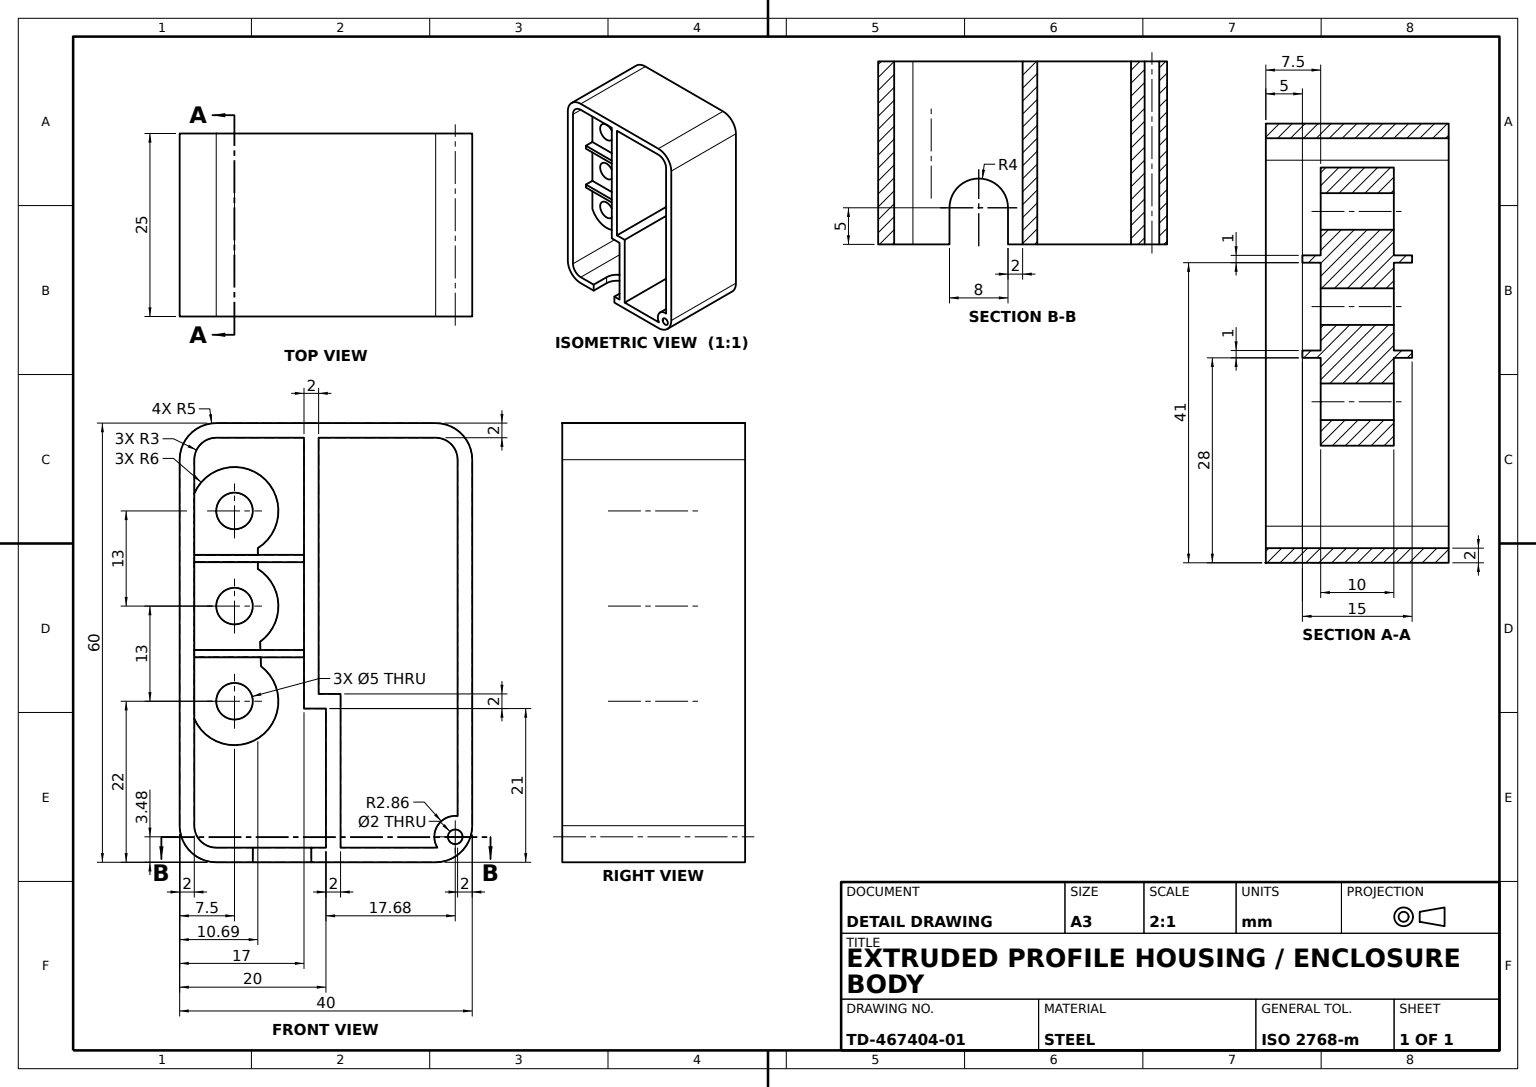
solid
v1 (-3,-9,12.5)
v2 (-3,-9,-12.5)
e1 v1 v2 LINE
v3 (0,-9,-12.5)
e2 v2 v3 LINE
v4 (0,-9,12.5)
e3 v4 v3 LINE
e4 v1 v4 LINE
face PLANE(AX(P(0,-9,12.5),D(0,1,0),D(0,0,1))) rev [e1 e2 -e3 -e4]
v5 (-10,-30,7.5)
v6 (-10,-30,12.5)
e5 v5 v6 LINE
v7 (-10,-28,7.5)
e6 v7 v5 LINE
v8 (-10,-28,12.5)
e7 v7 v8 LINE
e8 v8 v6 LINE
face PLANE(AX(P(-10,-30.000012,0),D(-1,0,0),D(0,0,1))) rev [-e5 -e6 e7 e8]
v9 (-9.3124,12.915793,5)
v10 (-18,20.396936,5)
e9 v9 v10 CIRCLE(AX(P(-12.5,17.99902,5),D(0,0,1),D(1,0,0)),6)
v11 (-18,11.99902,5)
e10 v10 v11 LINE
v12 (-9.3124,11.99902,5)
e11 v11 v12 LINE
e12 v9 v12 LINE
v13 (-10,17.99902,5)
v14 (-15,17.99902,5)
e13 v13 v14 CIRCLE(AX(P(-12.5,17.99902,5),D(0,0,1),D(1,0,0)),2.5)
e14 v14 v13 CIRCLE(AX(P(-12.5,17.99902,5),D(0,0,1),D(1,0,0)),2.5)
face PLANE(AX(P(0,0,5),D(0,0,1),D(1,0,0))) [e9 e10 e11 -e12] [-e13 -e14]
v15 (-10,4.99902,5)
v16 (-15,4.99902,5)
e15 v15 v16 CIRCLE(AX(P(-12.5,4.99902,5),D(0,0,1),D(1,0,0)),2.5)
e16 v16 v15 CIRCLE(AX(P(-12.5,4.99902,5),D(0,0,1),D(1,0,0)),2.5)
v17 (-9.3124,10.99902,5)
v18 (-9.3124,10.082248,5)
e17 v17 v18 LINE
v19 (-18,10.99902,5)
e18 v19 v17 LINE
v20 (-18,-1.00098,5)
e19 v19 v20 LINE
v21 (-8.958313,-1.00098,5)
e20 v20 v21 LINE
v22 (-8.994852,0.129325,5)
e21 v22 v21 LINE
e22 v22 v18 CIRCLE(AX(P(-12.5,4.99902,5),D(0,0,1),D(1,0,0)),6)
face PLANE(AX(P(0,0,5),D(0,0,1),D(1,0,0))) [-e15 -e16] [-e17 -e18 e19 e20 -e21 e22]
v23 (-6,-28,3.5)
v24 (-6,-30,3.5)
e23 v23 v24 LINE
v25 (-2,-30,7.5)
e24 v25 v24 CIRCLE(AX(P(-6,-30,7.5),D(0,1,0),D(0,0,-1)),4)
v26 (-2,-28,7.5)
e25 v26 v25 LINE
e26 v23 v26 CIRCLE(AX(P(-6,-28,7.5),D(0,-1,0),D(0,0,1)),4)
face CYL(AX(P(-6,-26,7.5),D(0,-1,0),D(0,0,-1)),4) rev [e23 -e24 -e25 -e26]
v27 (-3,-1.00098,7.5)
v28 (-3,-1.00098,-7.5)
e27 v27 v28 LINE
v29 (-18,-1.00098,-7.5)
e28 v29 v28 LINE
v30 (-18,-1.00098,-5)
e29 v30 v29 LINE
v31 (-8.958313,-1.00098,-5)
e30 v30 v31 LINE
e31 v21 v31 LINE
v32 (-18,-1.00098,7.5)
e32 v32 v20 LINE
e33 v32 v27 LINE
face PLANE(AX(P(0,-1.00098,7.5),D(0,1,0),D(0,0,1))) [e27 -e28 -e29 e30 -e31 -e20 -e32 e33]
v33 (-8.994852,0.129325,-5)
v34 (-9.3124,10.082248,-5)
e34 v33 v34 CIRCLE(AX(P(-12.5,4.99902,-5),D(0,0,1),D(1,0,0)),6)
e35 v18 v34 LINE
e36 v22 v33 LINE
face CYL(AX(P(-12.5,4.99902,5),D(0,0,-1),D(-1,0,0)),6) [e34 -e35 -e22 e36]
v35 (-18,10.99902,-5)
e37 v35 v30 LINE
v36 (-18,-2.00098,-7.5)
e38 v29 v36 LINE
v37 (-18,-2.00098,-5)
e39 v37 v36 LINE
v38 (-18,-10.398895,-5)
e40 v37 v38 LINE
v39 (-18,-10.398895,5)
e41 v39 v38 LINE
v40 (-18,-2.00098,5)
e42 v40 v39 LINE
v41 (-18,-2.00098,7.5)
e43 v41 v40 LINE
e44 v32 v41 LINE
v42 (-18,10.99902,7.5)
e45 v42 v19 LINE
v43 (-18,11.99902,7.5)
e46 v43 v42 LINE
e47 v43 v11 LINE
v44 (-18,20.396936,-5)
e48 v10 v44 LINE
v45 (-18,11.99902,-5)
e49 v44 v45 LINE
v46 (-18,11.99902,-7.5)
e50 v45 v46 LINE
v47 (-18,10.99902,-7.5)
e51 v46 v47 LINE
e52 v35 v47 LINE
v48 (-18,25,12.5)
v49 (-18,25,-12.5)
e53 v48 v49 LINE
v50 (-18,-25,12.5)
e54 v48 v50 LINE
v51 (-18,-25,-12.5)
e55 v50 v51 LINE
e56 v49 v51 LINE
face PLANE(AX(P(-18,0,12.5),D(1,0,0),D(0,1,0))) [e37 e29 e38 -e39 e40 -e41 -e42 -e43 -e44 e32 -e19 -e45 -e46 e47 -e10 e48 e49 e50 e51 -e52] [-e53 e54 e55 -e56]
v52 (-2,-28,12.5)
e57 v52 v26 LINE
v53 (0,-28,12.5)
e58 v52 v53 LINE
v54 (0,-28,-12.5)
e59 v53 v54 LINE
v55 (-15,-28,-12.5)
e60 v55 v54 LINE
v56 (-15,-28,12.5)
e61 v56 v55 LINE
e62 v56 v8 LINE
e63 v7 v23 CIRCLE(AX(P(-6,-28,7.5),D(0,-1,0),D(0,0,1)),4)
face PLANE(AX(P(0,-28,12.5),D(0,1,0),D(0,0,1))) [e26 -e57 e58 e59 -e60 -e61 e62 -e7 e63]
v57 (-3,-2.00098,7.5)
e64 v41 v57 LINE
e65 v27 v57 LINE
face PLANE(AX(P(0,0,7.5),D(0,0,1),D(1,0,0))) [e44 e64 -e65 -e33]
v58 (15,30,12.5)
v59 (15,30,-12.5)
e66 v58 v59 LINE
v60 (-15,30,-12.5)
e67 v60 v59 LINE
v61 (-15,30,12.5)
e68 v61 v60 LINE
e69 v61 v58 LINE
face PLANE(AX(P(0,30,12.5),D(0,1,0),D(0,0,1))) [e66 -e67 -e68 e69]
v62 (18.679633,-26.51945,12.5)
v63 (18.679633,-26.51945,-12.5)
e70 v62 v63 LINE
v64 (16.679633,-26.51945,12.5)
e71 v62 v64 CIRCLE(AX(P(17.679633,-26.51945,12.5),D(0,0,1),D(1,0,0)),1)
v65 (16.679633,-26.51945,-12.5)
e72 v64 v65 LINE
e73 v63 v65 CIRCLE(AX(P(17.679633,-26.51945,-12.5),D(0,0,1),D(1,0,0)),1)
face CYL(AX(P(17.679633,-26.51945,12.5),D(0,0,-1),D(-1,0,0)),1) rev [-e70 e71 e72 -e73]
v66 (-15,17.99902,-5)
e74 v14 v66 LINE
v67 (-10,17.99902,-5)
e75 v13 v67 LINE
e76 v66 v67 CIRCLE(AX(P(-12.5,17.99902,-5),D(0,0,1),D(1,0,0)),2.5)
face CYL(AX(P(-12.5,17.99902,5),D(0,0,-1),D(-1,0,0)),2.5) rev [-e74 e14 e75 -e76]
v68 (-20,25,12.5)
v69 (-20,25,-12.5)
e77 v68 v69 LINE
v70 (-20,-25,-12.5)
e78 v69 v70 LINE
v71 (-20,-25,12.5)
e79 v71 v70 LINE
e80 v68 v71 LINE
face PLANE(AX(P(-20,0,12.5),D(1,0,0),D(0,1,0))) rev [e77 e78 -e79 -e80]
v72 (-8.886875,-3.210851,5)
v73 (-8.886875,-3.210851,-5)
e81 v72 v73 LINE
e82 v39 v72 CIRCLE(AX(P(-12.5,-8.00098,5),D(0,0,1),D(1,0,0)),6)
e83 v38 v73 CIRCLE(AX(P(-12.5,-8.00098,-5),D(0,0,1),D(1,0,0)),6)
face CYL(AX(P(-12.5,-8.00098,5),D(0,0,-1),D(-1,0,0)),6) [-e81 -e82 e41 e83]
v74 (-3,-2.00098,-7.5)
e84 v28 v74 LINE
e85 v36 v74 LINE
face PLANE(AX(P(0,0,-7.5),D(0,0,1),D(1,0,0))) rev [e28 e84 -e85 -e38]
v75 (14.8185,-26.51945,12.5)
v76 (14.8185,-26.51945,-12.5)
e86 v75 v76 LINE
v77 (15.231357,-28,-12.5)
e87 v76 v77 CIRCLE(AX(P(17.679633,-26.51945,-12.5),D(0,0,1),D(1,0,0)),2.861134)
v78 (15.231357,-28,12.5)
e88 v78 v77 LINE
e89 v75 v78 CIRCLE(AX(P(17.679633,-26.51945,12.5),D(0,0,1),D(1,0,0)),2.861134)
face CYL(AX(P(17.679633,-26.51945,12.5),D(0,0,-1),D(-1,0,0)),2.861134) [e86 e87 -e88 -e89]
v79 (-1,28,12.5)
v80 (-1,28,-12.5)
e90 v79 v80 LINE
v81 (15,28,-12.5)
e91 v80 v81 LINE
v82 (15,28,12.5)
e92 v82 v81 LINE
e93 v79 v82 LINE
face PLANE(AX(P(0,28,12.5),D(0,1,0),D(0,0,1))) rev [e90 e91 -e92 -e93]
e94 v60 v69 CIRCLE(AX(P(-15,25,-12.5),D(0,0,1),D(1,0,0)),5)
v83 (20,25,-12.5)
e95 v59 v83 CIRCLE(AX(P(15,25,-12.5),D(0,0,-1),D(1,0,0)),5)
v84 (20,-25,-12.5)
e96 v83 v84 LINE
v85 (15,-30,-12.5)
e97 v85 v84 CIRCLE(AX(P(15,-25,-12.5),D(0,0,1),D(1,0,0)),5)
v86 (-15,-30,-12.5)
e98 v86 v85 LINE
e99 v70 v86 CIRCLE(AX(P(-15,-25,-12.5),D(0,0,1),D(1,0,0)),5)
v87 (18,25,-12.5)
e100 v81 v87 CIRCLE(AX(P(15,25,-12.5),D(0,0,-1),D(1,0,0)),3)
v88 (-1,-7,-12.5)
e101 v80 v88 LINE
v89 (2,-7,-12.5)
e102 v88 v89 LINE
v90 (2,-28,-12.5)
e103 v89 v90 LINE
e104 v90 v77 LINE
v91 (18,-23.676309,-12.5)
e105 v91 v76 CIRCLE(AX(P(17.679633,-26.51945,-12.5),D(0,0,1),D(1,0,0)),2.861134)
e106 v87 v91 LINE
v92 (-15,28,-12.5)
v93 (-3,28,-12.5)
e107 v92 v93 LINE
e108 v92 v49 CIRCLE(AX(P(-15,25,-12.5),D(0,0,1),D(1,0,0)),3)
e109 v51 v55 CIRCLE(AX(P(-15,-25,-12.5),D(0,0,1),D(1,0,0)),3)
e110 v3 v54 LINE
e111 v93 v2 LINE
e112 v65 v63 CIRCLE(AX(P(17.679633,-26.51945,-12.5),D(0,0,1),D(1,0,0)),1)
face PLANE(AX(P(0,0,-12.5),D(0,0,1),D(1,0,0))) rev [-e78 -e94 e67 e95 e96 -e97 -e98 -e99] [-e100 -e91 e101 e102 e103 e104 -e87 -e105 -e106] [-e107 e108 e56 e109 e60 -e110 -e2 -e111] [e112 e73]
v94 (-9.3124,12.915793,-5)
e113 v9 v94 LINE
e114 v94 v44 CIRCLE(AX(P(-12.5,17.99902,-5),D(0,0,1),D(1,0,0)),6)
face CYL(AX(P(-12.5,17.99902,5),D(0,0,-1),D(-1,0,0)),6) [-e9 e113 e114 -e48]
v95 (20,25,12.5)
e115 v95 v83 LINE
e116 v58 v95 CIRCLE(AX(P(15,25,12.5),D(0,0,-1),D(1,0,0)),5)
face CYL(AX(P(15,25,12.5),D(0,0,-1),D(-1,0,0)),5) [e115 -e95 -e66 e116]
v96 (-8.925986,-2.00098,5)
v97 (-8.925986,-2.00098,-5)
e117 v96 v97 LINE
e118 v96 v72 LINE
e119 v97 v73 LINE
face PLANE(AX(P(-8.981286,-0.290334,5),D(0.999477908,0.032309627,0),D(-0.032309627,0.999477908,0))) [-e117 e118 e81 -e119]
e120 v40 v96 LINE
e121 v37 v97 LINE
e122 v57 v74 LINE
face PLANE(AX(P(0,-2.00098,7.5),D(0,1,0),D(0,0,1))) rev [e120 e117 -e121 e39 e85 -e122 -e64 e43]
e123 v64 v62 CIRCLE(AX(P(17.679633,-26.51945,12.5),D(0,0,1),D(1,0,0)),1)
v98 (18,25,12.5)
e124 v82 v98 CIRCLE(AX(P(15,25,12.5),D(0,0,-1),D(1,0,0)),3)
v99 (18,-23.676309,12.5)
e125 v98 v99 LINE
e126 v99 v75 CIRCLE(AX(P(17.679633,-26.51945,12.5),D(0,0,1),D(1,0,0)),2.861134)
v100 (2,-28,12.5)
e127 v100 v78 LINE
v101 (2,-7,12.5)
e128 v101 v100 LINE
v102 (-1,-7,12.5)
e129 v102 v101 LINE
e130 v79 v102 LINE
v103 (-15,28,12.5)
e131 v103 v48 CIRCLE(AX(P(-15,25,12.5),D(0,0,1),D(1,0,0)),3)
v104 (-3,28,12.5)
e132 v103 v104 LINE
e133 v104 v1 LINE
e134 v4 v53 LINE
v105 (-2,-30,12.5)
e135 v105 v52 LINE
v106 (15,-30,12.5)
e136 v105 v106 LINE
v107 (20,-25,12.5)
e137 v106 v107 CIRCLE(AX(P(15,-25,12.5),D(0,0,1),D(1,0,0)),5)
e138 v95 v107 LINE
e139 v61 v68 CIRCLE(AX(P(-15,25,12.5),D(0,0,1),D(1,0,0)),5)
v108 (-15,-30,12.5)
e140 v71 v108 CIRCLE(AX(P(-15,-25,12.5),D(0,0,1),D(1,0,0)),5)
e141 v108 v6 LINE
e142 v50 v56 CIRCLE(AX(P(-15,-25,12.5),D(0,0,1),D(1,0,0)),3)
face PLANE(AX(P(0,0,12.5),D(0,0,1),D(1,0,0))) [-e71 -e123] [e93 e124 e125 e126 e89 -e127 -e128 -e129 -e130] [-e131 e132 e133 e4 e134 -e58 -e135 e136 e137 -e138 -e116 -e69 e139 e80 e140 e141 -e8 -e62 -e142 -e54]
e143 v107 v84 LINE
face PLANE(AX(P(20,0,12.5),D(1,0,0),D(0,1,0))) [-e96 -e115 e138 e143]
e144 v106 v85 LINE
face CYL(AX(P(15,-25,12.5),D(0,0,-1),D(-1,0,0)),5) [-e137 e144 e97 -e143]
e145 v100 v90 LINE
e146 v101 v89 LINE
face PLANE(AX(P(2,0,12.5),D(1,0,0),D(0,1,0))) [e128 e145 -e103 -e146]
face CYL(AX(P(-15,-25,12.5),D(0,0,-1),D(-1,0,0)),3) rev [-e55 e142 e61 -e109]
v109 (-3,11.99902,7.5)
e147 v43 v109 LINE
v110 (-3,10.99902,7.5)
e148 v42 v110 LINE
e149 v109 v110 LINE
face PLANE(AX(P(0,0,7.5),D(0,0,1),D(1,0,0))) [-e147 e46 e148 -e149]
face PLANE(AX(P(0,-28,12.5),D(0,1,0),D(0,0,1))) [e127 e88 -e104 -e145]
e150 v24 v5 CIRCLE(AX(P(-6,-30,7.5),D(0,1,0),D(0,0,-1)),4)
e151 v108 v86 LINE
e152 v105 v25 LINE
face PLANE(AX(P(0,-30,12.5),D(0,1,0),D(0,0,1))) rev [e24 e150 e5 -e141 e151 e98 -e144 -e136 e152]
v111 (-15,-8.00098,-5)
v112 (-10,-8.00098,-5)
e153 v111 v112 CIRCLE(AX(P(-12.5,-8.00098,-5),D(0,0,1),D(1,0,0)),2.5)
e154 v112 v111 CIRCLE(AX(P(-12.5,-8.00098,-5),D(0,0,1),D(1,0,0)),2.5)
face PLANE(AX(P(0,0,-5),D(0,0,1),D(1,0,0))) rev [e153 e154] [e119 -e83 -e40 e121]
v113 (-3,11.99902,-7.5)
e155 v46 v113 LINE
v114 (-3,10.99902,-7.5)
e156 v113 v114 LINE
e157 v47 v114 LINE
face PLANE(AX(P(0,0,-7.5),D(0,0,1),D(1,0,0))) rev [-e51 e155 e156 -e157]
v115 (-10,-8.00098,5)
e158 v115 v112 LINE
v116 (-15,-8.00098,5)
e159 v115 v116 CIRCLE(AX(P(-12.5,-8.00098,5),D(0,0,1),D(1,0,0)),2.5)
e160 v116 v111 LINE
face CYL(AX(P(-12.5,-8.00098,5),D(0,0,-1),D(-1,0,0)),2.5) rev [-e158 e159 e160 -e154]
e161 v104 v93 LINE
e162 v110 v114 LINE
e163 v109 v113 LINE
face PLANE(AX(P(-3,0,12.5),D(1,0,0),D(0,1,0))) rev [-e1 -e133 e161 e111] [e149 e162 -e156 -e163] [-e27 e65 e122 -e84]
e164 v33 v31 LINE
face PLANE(AX(P(-8.981286,-0.290334,5),D(0.999477908,0.032309627,0),D(-0.032309627,0.999477908,0))) [e31 -e164 -e36 e21]
v117 (-9.3124,11.99902,-5)
e165 v45 v117 LINE
e166 v12 v117 LINE
face PLANE(AX(P(0,11.99902,7.5),D(0,1,0),D(0,0,1))) [-e11 -e47 e147 e163 -e155 -e50 e165 -e166]
e167 v99 v91 LINE
face CYL(AX(P(17.679633,-26.51945,12.5),D(0,0,-1),D(-1,0,0)),2.861134) [e105 -e86 -e126 e167]
face PLANE(AX(P(0,0,12.5),D(1,0,0),D(0,1,0))) rev [-e134 e3 e110 -e59]
face CYL(AX(P(-6,-26,7.5),D(0,-1,0),D(0,0,-1)),4) rev [-e150 -e23 -e63 e6]
e168 v116 v115 CIRCLE(AX(P(-12.5,-8.00098,5),D(0,0,1),D(1,0,0)),2.5)
face CYL(AX(P(-12.5,-8.00098,5),D(0,0,-1),D(-1,0,0)),2.5) rev [e158 -e153 -e160 e168]
v118 (-10,4.99902,-5)
v119 (-15,4.99902,-5)
e169 v118 v119 CIRCLE(AX(P(-12.5,4.99902,-5),D(0,0,1),D(1,0,0)),2.5)
e170 v119 v118 CIRCLE(AX(P(-12.5,4.99902,-5),D(0,0,1),D(1,0,0)),2.5)
v120 (-9.3124,10.99902,-5)
e171 v35 v120 LINE
e172 v120 v34 LINE
face PLANE(AX(P(0,0,-5),D(0,0,1),D(1,0,0))) rev [e169 e170] [-e37 e171 e172 -e34 e164 -e30]
e173 v94 v117 LINE
face PLANE(AX(P(-9.3124,0,5),D(1,0,0),D(0,0,-1))) [e166 -e173 -e113 e12]
e174 v17 v120 LINE
face PLANE(AX(P(-9.3124,0,5),D(1,0,0),D(0,0,-1))) [-e172 -e174 e17 e35]
e175 v98 v87 LINE
face PLANE(AX(P(18,0,12.5),D(1,0,0),D(0,1,0))) rev [-e167 -e125 e175 e106]
e176 v102 v88 LINE
face PLANE(AX(P(0,-7,12.5),D(0,1,0),D(-1,0,0))) [e129 e146 -e102 -e176]
face CYL(AX(P(15,25,12.5),D(0,0,-1),D(-1,0,0)),3) rev [-e175 -e124 e92 e100]
face CYL(AX(P(-15,-25,12.5),D(0,0,-1),D(-1,0,0)),5) [e99 -e151 -e140 e79]
face CYL(AX(P(-15,25,12.5),D(0,0,-1),D(-1,0,0)),5) [e68 e94 -e77 -e139]
face PLANE(AX(P(-2,-30.000012,0),D(1,0,0),D(0,0,-1))) rev [-e152 e135 e57 e25]
e177 v67 v66 CIRCLE(AX(P(-12.5,17.99902,-5),D(0,0,1),D(1,0,0)),2.5)
face PLANE(AX(P(0,0,-5),D(0,0,1),D(1,0,0))) rev [-e165 -e49 -e114 e173] [e177 e76]
e178 v103 v92 LINE
face CYL(AX(P(-15,25,12.5),D(0,0,-1),D(-1,0,0)),3) rev [e53 -e108 -e178 e131]
face PLANE(AX(P(-1,0,12.5),D(1,0,0),D(0,1,0))) [-e90 e130 e176 -e101]
face PLANE(AX(P(0,28,12.5),D(0,1,0),D(0,0,1))) rev [-e132 e178 e107 -e161]
face CYL(AX(P(17.679633,-26.51945,12.5),D(0,0,-1),D(-1,0,0)),1) rev [e123 e70 -e112 -e72]
e179 v16 v119 LINE
e180 v15 v118 LINE
face CYL(AX(P(-12.5,4.99902,5),D(0,0,-1),D(-1,0,0)),2.5) rev [-e179 e16 e180 -e170]
face CYL(AX(P(-12.5,4.99902,5),D(0,0,-1),D(-1,0,0)),2.5) rev [e179 -e169 -e180 e15]
face PLANE(AX(P(0,10.99902,7.5),D(0,1,0),D(0,0,1))) rev [-e148 e45 e18 e174 -e171 e52 e157 -e162]
face CYL(AX(P(-12.5,17.99902,5),D(0,0,-1),D(-1,0,0)),2.5) rev [e13 e74 -e177 -e75]
face PLANE(AX(P(0,0,5),D(0,0,1),D(1,0,0))) [-e159 -e168] [e42 e82 -e118 -e120]
